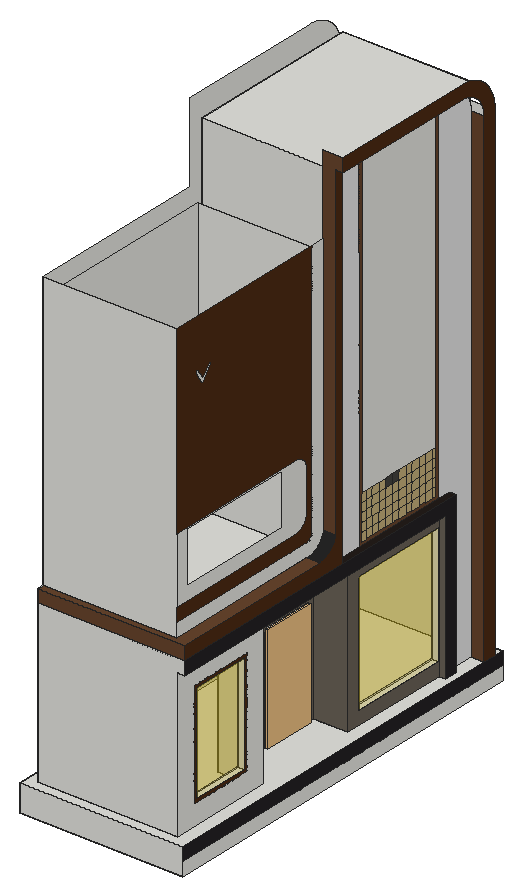
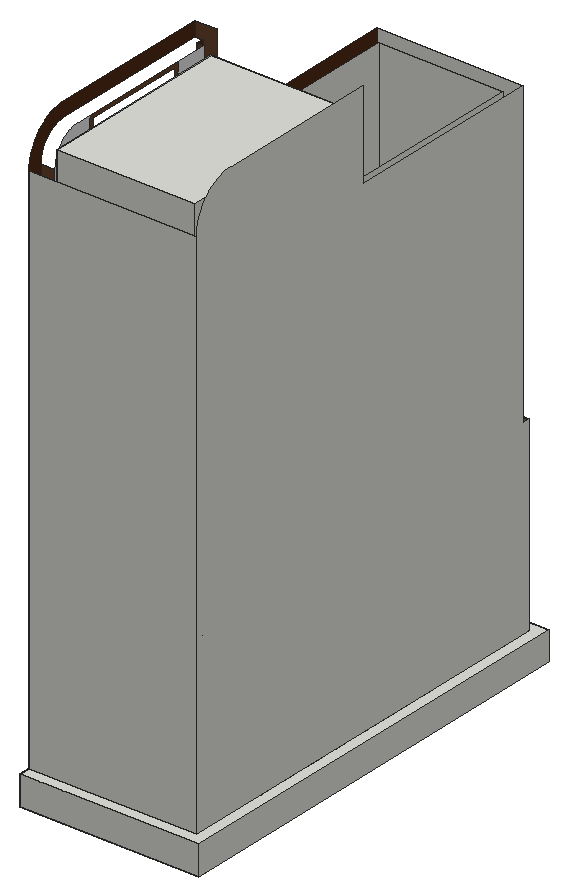
# SketchUp Ruby script. Lengths in inches.
U = 1.inch
M = Sketchup.active_model
def pt(a) = Geom::Point3d.new(a.map { |v| v * U })
def face(e, loops, mat)
  f = e.add_face(loops[0].map { |a| pt(a) })
  loops[1..].each { |l| e.add_face(l.map { |a| pt(a) }).erase! }
  f.material = f.back_material = mat if mat
  f
end
# faces: each face lists its corners as indices into pts; further lists are holes
def faces(e, pts, list, mat = nil) = list.each { |f| face(e, (f[0].is_a?(Array) ? f : [f]).map { |l| l.map { |i| pts[i] } }, mat) }
# xy, xz, yz: faces in a plane at the given z, y or x. An outline is a flat list of corners, or four numbers for a rectangle; further outlines are holes
def ring(l) = l.size == 4 ? [[l[0], l[1]], [l[2], l[1]], [l[2], l[3]], [l[0], l[3]]] : l.each_slice(2).to_a
def flat(e, list, mat, &to3) = list.each { |f| face(e, (f[0].is_a?(Array) ? f : [f]).map { |l| ring(l).map { |u, v| to3.(u, v) } }, mat) }
def xy(e, z, list, mat = nil) = flat(e, list, mat) { |x, y| [x, y, z] }
def xz(e, y, list, mat = nil) = flat(e, list, mat) { |x, z| [x, y, z] }
def yz(e, x, list, mat = nil) = flat(e, list, mat) { |y, z| [x, y, z] }
def lines(e, pts, list) = list.each { |a, b| e.add_line(pt(pts[a]), pt(pts[b])) }
# prism: a flat outline (further loops are holes) pulled along v
def prism(e, loops, v, mat = nil)
  f = face(e, loops, mat); d = Geom::Vector3d.new(v.map { |x| x * U })
  f.pushpull(f.normal.samedirection?(d) ? d.length : -d.length)
end
def box(e, o, s, mat = nil) = prism(e, [[o, [o[0] + s[0], o[1], o[2]], [o[0] + s[0], o[1] + s[1], o[2]], [o[0], o[1] + s[1], o[2]]]], [0, 0, s[2]], mat)
def at(x, y, z, deg = 0) = Geom::Transformation.translation(pt([x, y, z])) * Geom::Transformation.rotation(ORIGIN, Z_AXIS, deg.degrees)
def axes(o, x, y, z) = Geom::Transformation.new([*x, 0, *y, 0, *z, 0, *pt(o).to_a, 1])
def part(name) = M.definitions.add(name)
# library, detail: a bought-in or finely detailed component or shape, given as its bounding box
def library(name, o, s) = part(name).tap { |d| box(d.entities, o, s) }
def detail(e, o, s) = box(e.add_group.entities, o, s)
def put(e, d, t, mat = nil) = e.add_instance(d, t).tap { |i| i.material = mat if mat }
def group(e, t, mat = nil) = e.add_group.tap { |g| g.transformation = t; g.material = mat if mat }.entities
root = M.entities
M.materials.add("Glass_Basic_01").color = [255, 223, 26]
M.materials["Glass_Basic_01"].alpha = 0.25
M.materials.add("Marble_07_1K").color = [36, 34, 36]
M.materials.add("Metal_10_1K").color = [196, 175, 123]
M.materials.add("Plaster_04_1K").color = [106, 98, 87]
M.materials.add("Wood_Floor_12_1K").color = [35, 29, 25]
M.materials.add("Wood_Planks_01_1K").color = [69, 67, 63]
M.materials.add("Wood_Veneer_15_1K").color = [103, 69, 45]
M.materials.add("[Color_001]").color = [226, 226, 226]
M.materials.add("[Wood_Cherry_Original]1").color = [76, 43, 21]
c1 = library("porta+4",[0.2,-5.42,1.33],[46.55,4.72,83.21])
box(root,[15,186,177],[114,159,307.29])
xy(root,0,[[0,0,147,360]])
xy(root,24,[[0,0,147,0,147,339,135,339,135,315,141,315,141,303,135,303,135,201,103.5,201,103.5,105,135,105,135,9,9,9,9,351,147,351,147,360,0,360],[9,9,135,9,135,105,129,105,129,15,15,15,15,291,9,291],[15,15,129,15,129,99,99,99,99,207,129,207,129,345,15,345],[99,99,129,99,129,105,103.5,105,103.5,201,135,201,135,291,129,291,129,207,99,207],[9,291,15,291,15,345,129,345,129,291,135,291,135,339,147,339,147,351,9,351]])
xy(root,27,[[99,150,103.5,192]])
xy(root,36,[[129,213,135,303]])
xy(root,45,[[129,30,135,84]])
xy(root,117,[[99,150,103.5,192]])
xy(root,135,[[129,30,135,84]])
xy(root,144,[[129,213,135,303]])
xy(root,156,[[135,9,135,105,103.5,105,103.5,201,135,201,135,303,141,303,141,9]],"Plaster_04_1K")
xy(root,168,[[9,9,129,15],[15,15,15,345,129,345,129,207,99,207,99,99,129,99,129,15]])
xy(root,168,[[135,186,141,315]],"Wood_Floor_12_1K")
xy(root,177,[[21,21,123,174]])
xy(root,180,[[9,9,141,9,141,162,129,162,129,15,9,15],[129,162,141,162.25]],"Wood_Veneer_15_1K")
xz(root,0,[[0,0,147,24]])
xz(root,9,[[9,24,135,24,135,156,141,156,141,168,9,168]])
xz(root,9,[[9,168,141,180]],"Wood_Veneer_15_1K")
xz(root,15,[[15,24,129,168],[9,180,129,429]])
xz(root,21,[[21,177,123,423]])
xz(root,30,[[129,45,135,135]])
xz(root,84,[[129,45,135,135]])
xz(root,99,[[99,24,129,168]])
xz(root,105,[[103.5,24,135,156]])
xz(root,150,[[99,27,103.5,117]])
xz(root,174,[[21,177,123,423]])
xz(root,180,[[129,194.38,141,194.38,141,489,147,489,147,501,129,501]],"Wood_Veneer_15_1K")
xz(root,186,[[135,168,141,170],[135,170,141,170.38],[135,170.38,141,489]],"Wood_Veneer_15_1K")
xz(root,192,[[99,27,103.5,117]])
xz(root,201,[[103.5,24,135,156]],"Plaster_04_1K")
xz(root,207,[[99,24,129,168]])
xz(root,213,[[129,36,135,144]])
xz(root,303,[[129,36,135,144]])
xz(root,303,[[135,24,141,156]],"Plaster_04_1K")
xz(root,315,[[135,24,141,168]],"Wood_Floor_12_1K")
xz(root,339,[[135,24,147,465]],"Wood_Veneer_15_1K")
xz(root,345,[[15,24,129,168]])
xz(root,351,[[9,24,147,465]])
xz(root,360,[[0,0,147,24]])
yz(root,0,[[0,0,360,24]])
yz(root,9,[[9,24,9,180,15,180,15,429,180,429,180,501,315,501,316.13,500.98,317.26,500.93,318.39,500.84,319.51,500.72,320.63,500.56,321.75,500.36,322.85,500.13,323.95,499.87,325.04,499.57,326.125,499.24,327.19,498.87,328.25,498.47,329.3,498.04,330.33,497.57,331.34,497.08,332.34,496.55,333.33,495.99,334.29,495.4,335.24,494.77,336.16,494.125,337.06,493.45,337.95,492.74,338.81,492,339.64,491.24,340.46,490.46,341.24,489.64,342,488.81,342.74,487.95,343.45,487.06,344.125,486.16,344.77,485.24,345.4,484.29,345.99,483.33,346.55,482.34,347.08,481.34,347.57,480.33,348.04,479.3,348.47,478.25,348.87,477.19,349.24,476.125,349.57,475.04,349.87,473.95,350.13,472.85,350.36,471.75,350.56,470.63,350.72,469.51,350.84,468.39,350.93,467.26,350.98,466.13,351,465,351,24]])
yz(root,15,[[15,24,345,168]])
yz(root,21,[[21,177,174,423]])
yz(root,99,[[[99,24,207,168],[150,27,192,117]]])
yz(root,103.5,[[[147,24,195,120],[150,27,192,117]]])
yz(root,103.5,[[105,24,147,24,147,120,195,120,195,24,201,24,201,156,105,156]],"Plaster_04_1K")
yz(root,123,[[[21,177,174,423],[34,211,140.71,257]]])
yz(root,129,[[[15,24,99,168],[30,45,84,135]],[[207,24,345,168],[213,36,303,144]],[15,180,162.25,180,162.75,180.02,162.99,180.03,163.24,180.04,163.74,180.08,163.99,180.11,164.23,180.14,164.73,180.2,164.97,180.24,165.22,180.28,165.46,180.33,165.71,180.375,165.95,180.43,166.19,180.48,166.43,180.54,166.68,180.6,166.92,180.67,167.16,180.73,167.39,180.81,167.63,180.88,167.87,180.96,168.1,181.04,168.34,181.12,169.03,181.39,169.72,181.69,169.94,181.8,170.17,181.9,170.39,182.02,170.61,182.13,171.05,182.37,171.26,182.49,171.48,182.62,171.6875,182.75,171.9,182.88,172.11,183.01,172.32,183.15,172.52,183.29,172.73,183.4375,172.93,183.58,173.32,183.88,173.52,184.04,173.71,184.19,174.09,184.51,174.28,184.68,174.46,184.84,174.65,185.01,174.83,185.1875,175,185.36,175.35,185.71,175.52,185.9,175.69,186.08,175.86,186.27,176.02,186.45,176.18,186.64,176.34,186.84,176.49,187.03,176.65,187.23,176.8,187.42,176.94,187.625,177.09,187.83,177.23,188.03,177.51,188.45,177.9,189.08,178.02,189.3,178.14,189.51,178.38,189.95,178.49,190.17,178.6,190.4,178.71,190.62,178.8125,190.85,178.92,191.07,179.01,191.3,179.11,191.53,179.2,191.76,179.29,192,179.375,192.23,179.46,192.47,179.54,192.7,179.61,192.9375,179.68,193.18,179.75,193.41,179.82,193.65,179.88,193.9,180,194.38,180,429,168,429,168,196.07,167.98,196.03,167.95,195.95,167.92,195.875,167.88,195.79,167.85,195.72,167.73,195.48,167.6875,195.4,167.65,195.33,167.6,195.25,167.5625,195.18,167.52,195.1,167.47,195.03,167.42,194.95,167.33,194.81,167.18,194.6,167.07,194.46,167.02,194.39,166.96,194.32,166.9,194.26,166.85,194.19,166.79,194.125,166.49,193.8125,166.42,193.75,166.36,193.69,166.3,193.64,166.16,193.52,166.1,193.47,166.03,193.41,165.89,193.31,165.82,193.25,165.54,193.05,165.46,193.01,165.39,192.96,165.31,192.92,165.24,192.87,165.16,192.83,165.09,192.79,164.93,192.71,164.86,192.67,164.7,192.59,164.62,192.56,164.54,192.52,164.46,192.49,164.38,192.45,164.22,192.39,164.13,192.36,164.05,192.34,163.89,192.28,163.8,192.26,163.72,192.23,163.55,192.1875,163.47,192.17,163.38,192.15,163.3,192.13,163.21,192.11,163.125,192.1,163.04,192.08,162.95,192.07,162.87,192.06,162.69,192.04,162.61,192.03,162.43,192.01,162.26,192.01,162.17,192,15,192]])
yz(root,129,[[213,36,303,144],[30,45,84,135]],"Glass_Basic_01")
yz(root,129,[[[15,192,162.17,192,162.26,192.01,162.43,192.01,162.61,192.03,162.69,192.04,162.87,192.06,162.95,192.07,163.04,192.08,163.125,192.1,163.21,192.11,163.3,192.13,163.38,192.15,163.47,192.17,163.55,192.1875,163.72,192.23,163.8,192.26,163.89,192.28,164.05,192.34,164.13,192.36,164.22,192.39,164.38,192.45,164.46,192.49,164.54,192.52,164.62,192.56,164.7,192.59,164.86,192.67,164.93,192.71,165.09,192.79,165.16,192.83,165.24,192.87,165.31,192.92,165.39,192.96,165.46,193.01,165.54,193.05,165.82,193.25,165.89,193.31,166.03,193.41,166.1,193.47,166.16,193.52,166.3,193.64,166.36,193.69,166.42,193.75,166.49,193.8125,166.79,194.125,166.85,194.19,166.9,194.26,166.96,194.32,167.02,194.39,167.07,194.46,167.18,194.6,167.33,194.81,167.42,194.95,167.47,195.03,167.52,195.1,167.5625,195.18,167.6,195.25,167.65,195.33,167.6875,195.4,167.73,195.48,167.85,195.72,167.88,195.79,167.92,195.875,167.95,195.95,167.98,196.03,168,196.07,168,429,15,429,15,264,150.15,264,150.34,263.99,150.52,263.99,150.71,263.98,150.9,263.96,151.09,263.95,151.28,263.93,151.46,263.91,151.84,263.85,152.02,263.82,152.21,263.79,152.39,263.75,152.58,263.71,152.76,263.67,152.94,263.62,153.31,263.52,153.49,263.47,153.85,263.35,154.02,263.29,154.2,263.23,154.38,263.16,154.55,263.09,154.73,263.01,154.9,262.9375,155.07,262.86,155.24,262.78,155.41,262.69,155.57,262.61,155.74,262.52,155.91,262.42,156.07,262.33,156.55,262.03,156.7,261.92,156.86,261.82,157.16,261.6,157.3125,261.48,157.46,261.37,157.61,261.25,157.75,261.125,157.9,261,158.04,260.875,158.17,260.75,158.3125,260.62,158.44,260.49,158.58,260.35,158.71,260.21,158.84,260.08,158.96,259.9375,159.08,259.79,159.21,259.65,159.32,259.5,159.44,259.35,159.56,259.21,159.67,259.05,159.78,258.9,159.88,258.75,159.99,258.59,160.29,258.11,160.38,257.95,160.48,257.78,160.56,257.62,160.74,257.28,160.82,257.11,160.9,256.9375,160.97,256.77,161.05,256.59,161.12,256.42,161.18,256.24,161.25,256.06,161.3125,255.89,161.37,255.71,161.43,255.53,161.53,255.17,161.58,254.98,161.63,254.8,161.67,254.62,161.71,254.43,161.75,254.25,161.78,254.0625,161.8125,253.88,161.84,253.69,161.86,253.5,161.89,253.32,161.91,253.13,161.92,252.94,161.9375,252.75,161.95,252.57,161.95,252.375,161.96,252.1875,161.96,215.8125,161.95,215.625,161.95,215.43,161.9375,215.25,161.92,215.06,161.91,214.87,161.89,214.68,161.86,214.5,161.84,214.31,161.8125,214.12,161.78,213.9375,161.75,213.75,161.71,213.57,161.67,213.38,161.63,213.2,161.58,213.02,161.53,212.83,161.43,212.47,161.37,212.29,161.3125,212.11,161.25,211.94,161.18,211.76,161.12,211.58,161.05,211.41,160.97,211.23,160.9,211.0625,160.82,210.89,160.74,210.72,160.56,210.38,160.48,210.22,160.38,210.05,160.29,209.89,159.99,209.41,159.88,209.25,159.78,209.1,159.67,208.95,159.56,208.79,159.44,208.65,159.32,208.5,159.21,208.35,159.08,208.21,158.96,208.0625,158.84,207.92,158.71,207.79,158.58,207.65,158.44,207.51,158.3125,207.38,158.17,207.25,158.04,207.125,157.9,207,157.75,206.875,157.61,206.75,157.46,206.63,157.3125,206.52,157.16,206.4,156.86,206.18,156.7,206.08,156.55,205.97,156.07,205.67,155.91,205.58,155.74,205.48,155.57,205.39,155.41,205.31,155.24,205.22,155.07,205.14,154.9,205.0625,154.73,204.99,154.55,204.91,154.38,204.84,154.2,204.77,154.02,204.71,153.85,204.65,153.49,204.53,153.31,204.48,152.94,204.38,152.76,204.33,152.58,204.29,152.39,204.25,152.21,204.21,152.02,204.18,151.84,204.15,151.46,204.09,151.28,204.07,151.09,204.05,150.9,204.04,150.71,204.02,150.52,204.01,150.34,204.01,150.15,204,15,204],[45.07,371.33,42.96,374.22,43.02,374.3,36.28,383.51,36.24,383.87,36.27,384.22,36.36,384.57,36.52,384.89,36.74,385.17,37,385.41,37.3125,385.59,37.65,385.72,38,385.77,38.36,385.75,38.71,385.67,39.03,385.52,45.13,377.19,51.23,385.52,51.56,385.67,51.9,385.75,52.26,385.77,52.62,385.72,52.95,385.59,53.26,385.41,53.53,385.17,53.74,384.89,53.9,384.57,54,384.22,54.02,383.87,53.98,383.51,47.18,374.22,45.26,371.58]]],"[Wood_Cherry_Original]1")
yz(root,135,[[[9,24,105,156],[27,42,87,138]]])
yz(root,135,[[213,36,303,144],[30,45,84,135]],"Glass_Basic_01")
yz(root,135,[[216,171,220.5,178.875],[220.5,171,228,178.875],[228,171,235.5,178.875],[235.5,171,243,178.875],[243,171,250.5,178.875],
  [250.5,171,258,178.875],[258,171,265.5,178.875],[265.5,171,273,178.875],[273,171,280.5,178.875],[280.5,171,288,178.875],
  [288,171,295.5,178.875],[295.5,171,300,178.875],[216,178.875,220.5,186.75],[220.5,178.875,228,186.75],[228,178.875,235.5,186.75],
  [235.5,178.875,243,186.75],[243,178.875,250.5,186.75],[250.5,178.875,258,186.75],[258,178.875,265.5,186.75],[265.5,178.875,273,186.75],
  [273,178.875,280.5,186.75],[280.5,178.875,288,186.75],[288,178.875,295.5,186.75],[295.5,178.875,300,186.75],[216,186.75,220.5,194.625],
  [220.5,186.75,228,194.625],[228,186.75,235.5,194.625],[235.5,186.75,243,194.625],[243,186.75,250.5,194.625],[250.5,186.75,258,194.625],
  [258,186.75,265.5,194.625],[265.5,186.75,273,194.625],[273,186.75,280.5,194.625],[280.5,186.75,288,194.625],[288,186.75,295.5,194.625],
  [295.5,186.75,300,194.625],[216,194.625,220.5,202.5],[220.5,194.625,228,202.5],[228,194.625,235.5,202.5],[235.5,194.625,243,202.5],
  [243,194.625,250.5,202.5],[250.5,194.625,258,202.5],[258,194.625,265.5,202.5],[265.5,194.625,273,202.5],[273,194.625,280.5,202.5],
  [280.5,194.625,288,202.5],[288,194.625,295.5,202.5],[295.5,194.625,300,202.5],[216,202.5,220.5,210.375],[220.5,202.5,228,210.375],
  [228,202.5,235.5,210.375],[235.5,202.5,243,210.375],[258,202.5,265.5,210.375],[265.5,202.5,273,210.375],[273,202.5,280.5,210.375],
  [280.5,202.5,288,210.375],[288,202.5,295.5,210.375],[295.5,202.5,300,210.375]],"Metal_10_1K")
yz(root,135,[[201,24,303,24,303,36,213,36,213,144,303,144,303,156,201,156]],"Plaster_04_1K")
yz(root,135,[[243,202.5,250.5,210.375],[250.5,202.5,258,210.375]],"Wood_Planks_01_1K")
yz(root,135,[[[213,168,303,489],[216,171,300,486]]],"Wood_Veneer_15_1K")
yz(root,135,[[315,24,339,24,339,465,338.99,465.75,338.95,466.51,338.89,467.26,338.8125,468.01,338.7,468.75,338.57,469.5,338.42,470.24,338.25,470.97,338.05,471.7,337.83,472.42,337.58,473.13,337.31,473.83,337.03,474.53,336.72,475.22,336.38,475.9,336.03,476.5625,335.66,477.22,335.26,477.86,334.85,478.49,334.42,479.11,333.96,479.71,333.49,480.3,333,480.87,332.5,481.43,331.97,481.97,331.43,482.5,330.87,483,330.3,483.49,329.71,483.96,329.11,484.42,328.49,484.85,327.86,485.26,327.22,485.66,326.5625,486.03,325.9,486.38,325.22,486.72,324.53,487.03,323.83,487.31,323.13,487.58,322.42,487.83,321.7,488.05,320.97,488.25,320.24,488.42,319.5,488.57,318.75,488.7,318.01,488.8125,317.26,488.89,316.51,488.95,315.75,488.99,315,489,303,489,303,168,315,168],[186,168,213,489]],"[Color_001]")
yz(root,135,[[[27,42,87,138],[30,45,84,135]]],"[Wood_Cherry_Original]1")
yz(root,141,[[303,24,315,24,315,168,9,168,9,156,303,156]],"Marble_07_1K")
yz(root,141,[[9,168,186,168,186,489,180,489,180,194.38,179.88,193.9,179.82,193.65,179.75,193.41,179.68,193.18,179.61,192.9375,179.54,192.7,179.46,192.47,179.375,192.23,179.29,192,179.2,191.76,179.11,191.53,179.01,191.3,178.92,191.07,178.8125,190.85,178.71,190.62,178.6,190.4,178.49,190.17,178.38,189.95,178.14,189.51,178.02,189.3,177.9,189.08,177.51,188.45,177.23,188.03,177.09,187.83,176.94,187.625,176.8,187.42,176.65,187.23,176.49,187.03,176.34,186.84,176.18,186.64,176.02,186.45,175.86,186.27,175.69,186.08,175.52,185.9,175.35,185.71,175,185.36,174.83,185.1875,174.65,185.01,174.46,184.84,174.28,184.68,174.09,184.51,173.71,184.19,173.52,184.04,173.32,183.88,172.93,183.58,172.73,183.4375,172.52,183.29,172.32,183.15,172.11,183.01,171.9,182.88,171.6875,182.75,171.48,182.62,171.26,182.49,171.05,182.37,170.61,182.13,170.39,182.02,170.17,181.9,169.94,181.8,169.72,181.69,169.03,181.39,168.34,181.12,168.1,181.04,167.87,180.96,167.63,180.88,167.39,180.81,167.16,180.73,166.92,180.67,166.68,180.6,166.43,180.54,166.19,180.48,165.95,180.43,165.71,180.375,165.46,180.33,165.22,180.28,164.97,180.24,164.73,180.2,164.23,180.14,163.99,180.11,163.74,180.08,163.24,180.04,162.99,180.03,162.75,180.02,162.25,180,9,180]],"[Wood_Cherry_Original]1")
yz(root,147,[[0,0,360,12]])
yz(root,147,[[0,12,360,24]],"Marble_07_1K")
yz(root,147,[[339,24,351,24,351,465,350.98,466.13,350.93,467.26,350.84,468.39,350.72,469.51,350.56,470.63,350.36,471.75,350.13,472.85,349.87,473.95,349.57,475.04,349.24,476.125,348.87,477.19,348.47,478.25,348.04,479.3,347.57,480.33,347.08,481.34,346.55,482.34,345.99,483.33,345.4,484.29,344.77,485.24,344.125,486.16,343.45,487.06,342.74,487.95,342,488.81,341.24,489.64,340.46,490.46,339.64,491.24,338.81,492,337.95,492.74,337.06,493.45,336.16,494.125,335.24,494.77,334.29,495.4,333.33,495.99,332.34,496.55,331.34,497.08,330.33,497.57,329.3,498.04,328.25,498.47,327.19,498.87,326.125,499.24,325.04,499.57,323.95,499.87,322.85,500.13,321.75,500.36,320.63,500.56,319.51,500.72,318.39,500.84,317.26,500.93,316.13,500.98,315,501,180,501,180,489,315,489,315.75,488.99,316.51,488.95,317.26,488.89,318.01,488.8125,318.75,488.7,319.5,488.57,320.24,488.42,320.97,488.25,321.7,488.05,322.42,487.83,323.13,487.58,323.83,487.31,324.53,487.03,325.22,486.72,325.9,486.38,326.5625,486.03,327.22,485.66,327.86,485.26,328.49,484.85,329.11,484.42,329.71,483.96,330.3,483.49,330.87,483,331.43,482.5,331.97,481.97,332.5,481.43,333,480.87,333.49,480.3,333.96,479.71,334.42,479.11,334.85,478.49,335.26,477.86,335.66,477.22,336.03,476.5625,336.38,475.9,336.72,475.22,337.03,474.53,337.31,473.83,337.58,473.13,337.83,472.42,338.05,471.7,338.25,470.97,338.42,470.24,338.57,469.5,338.7,468.75,338.8125,468.01,338.89,467.26,338.95,466.51,338.99,465.75,339,465]],"[Wood_Cherry_Original]1")
p = [[129,162.25,180],[141,162.25,180],[141,162.5,180.01],[129,162.5,180.01],[141,162.75,180.02],[129,162.75,180.02],
  [141,162.99,180.03],[129,162.99,180.03],[141,163.24,180.04],[129,163.24,180.04],[141,163.49,180.06],[129,163.49,180.06],
  [141,163.74,180.08],[129,163.74,180.08],[141,163.99,180.11],[129,163.99,180.11],[141,164.23,180.14],[129,164.23,180.14],
  [141,164.48,180.17],[129,164.48,180.17],[141,164.73,180.2],[129,164.73,180.2],[141,164.97,180.24],[129,164.97,180.24],
  [141,165.22,180.28],[129,165.22,180.28],[141,165.46,180.33],[129,165.46,180.33],[141,165.71,180.375],[129,165.71,180.375],
  [141,165.95,180.43],[129,165.95,180.43],[141,166.19,180.48],[129,166.19,180.48],[141,166.43,180.54],[129,166.43,180.54],
  [141,166.68,180.6],[129,166.68,180.6],[141,166.92,180.67],[129,166.92,180.67],[141,167.16,180.73],[129,167.16,180.73],
  [141,167.39,180.81],[129,167.39,180.81],[141,167.63,180.88],[129,167.63,180.88],[141,167.87,180.96],[129,167.87,180.96],
  [141,168.1,181.04],[129,168.1,181.04],[141,168.34,181.12],[129,168.34,181.12],[141,168.57,181.21],[129,168.57,181.21],
  [141,168.8,181.3],[129,168.8,181.3],[141,169.03,181.39],[129,169.03,181.39],[141,169.26,181.49],[129,169.26,181.49],
  [141,169.49,181.59],[129,169.49,181.59],[141,169.72,181.69],[129,169.72,181.69],[141,169.94,181.8],[129,169.94,181.8],
  [141,170.17,181.9],[129,170.17,181.9],[141,170.39,182.02],[129,170.39,182.02],[141,170.61,182.13],[129,170.61,182.13],
  [141,170.83,182.25],[129,170.83,182.25],[141,171.05,182.37],[129,171.05,182.37],[141,171.26,182.49],[129,171.26,182.49],
  [141,171.48,182.62],[129,171.48,182.62],[141,171.6875,182.75],[129,171.6875,182.75],[141,171.9,182.88],[129,171.9,182.88],
  [141,172.11,183.01],[129,172.11,183.01],[141,172.32,183.15],[129,172.32,183.15],[141,172.52,183.29],[129,172.52,183.29],
  [141,172.73,183.4375],[129,172.73,183.4375],[141,172.93,183.58],[129,172.93,183.58],[141,173.125,183.73],[129,173.125,183.73],
  [141,173.32,183.88],[129,173.32,183.88],[141,173.52,184.04],[129,173.52,184.04],[141,173.71,184.19],[129,173.71,184.19],
  [141,173.9,184.35],[129,173.9,184.35],[141,174.09,184.51],[129,174.09,184.51],[141,174.28,184.68],[129,174.28,184.68],
  [141,174.46,184.84],[129,174.46,184.84],[141,174.65,185.01],[129,174.65,185.01],[141,174.83,185.1875],[129,174.83,185.1875],
  [141,175,185.36],[129,175,185.36],[141,175.18,185.54],[129,175.18,185.54],[141,175.35,185.71],[129,175.35,185.71],
  [141,175.52,185.9],[129,175.52,185.9],[141,175.69,186.08],[129,175.69,186.08],[141,175.86,186.27],[129,175.86,186.27],
  [141,176.02,186.45],[129,176.02,186.45],[141,176.18,186.64],[129,176.18,186.64],[141,176.34,186.84],[129,176.34,186.84],
  [141,176.49,187.03],[129,176.49,187.03],[141,176.65,187.23],[129,176.65,187.23],[141,176.8,187.42],[129,176.8,187.42],
  [141,176.94,187.625],[129,176.94,187.625],[141,177.09,187.83],[129,177.09,187.83],[141,177.23,188.03],[129,177.23,188.03],
  [141,177.37,188.24],[129,177.37,188.24],[141,177.51,188.45],[129,177.51,188.45],[141,177.64,188.66],[129,177.64,188.66],
  [141,177.77,188.87],[129,177.77,188.87],[141,177.9,189.08],[129,177.9,189.08],[141,178.02,189.3],[129,178.02,189.3],
  [141,178.14,189.51],[129,178.14,189.51],[141,178.26,189.73],[129,178.26,189.73],[141,178.38,189.95],[129,178.38,189.95],
  [141,178.49,190.17],[129,178.49,190.17],[141,178.6,190.4],[129,178.6,190.4],[141,178.71,190.62],[129,178.71,190.62],
  [141,178.8125,190.85],[129,178.8125,190.85],[141,178.92,191.07],[129,178.92,191.07],[141,179.01,191.3],[129,179.01,191.3],
  [141,179.11,191.53],[129,179.11,191.53],[141,179.2,191.76],[129,179.2,191.76],[141,179.29,192],[129,179.29,192],
  [141,179.375,192.23],[129,179.375,192.23],[141,179.46,192.47],[129,179.46,192.47],[141,179.54,192.7],[129,179.54,192.7],
  [141,179.61,192.9375],[129,179.61,192.9375],[141,179.68,193.18],[129,179.68,193.18],[141,179.75,193.41],[129,179.75,193.41],
  [141,179.82,193.65],[129,179.82,193.65],[141,179.88,193.9],[129,179.88,193.9],[141,179.94,194.14],[129,179.94,194.14],
  [141,180,194.38],[129,180,194.38],[9,291,0],[9,291,24],[9,9,0],[9,9,24],
  [15,345,168],[9,345,168],[129,99,168],[129,105,168],[129,180,180],[135,180,180],
  [129,162,180]]
faces(root,p,[[0,1,2,3],[3,2,4,5],[5,4,6,7],[7,6,8,9],[9,8,10,11],[11,10,12,13],[13,12,14,15],[15,14,16,17],
  [17,16,18,19],[19,18,20,21],[21,20,22,23],[23,22,24,25],[25,24,26,27],[27,26,28,29],[29,28,30,31],[31,30,32,33],
  [33,32,34,35],[35,34,36,37],[37,36,38,39],[39,38,40,41],[41,40,42,43],[43,42,44,45],[45,44,46,47],[47,46,48,49],
  [49,48,50,51],[51,50,52,53],[53,52,54,55],[55,54,56,57],[57,56,58,59],[59,58,60,61],[61,60,62,63],[63,62,64,65],
  [65,64,66,67],[67,66,68,69],[69,68,70,71],[71,70,72,73],[73,72,74,75],[75,74,76,77],[77,76,78,79],[79,78,80,81],
  [81,80,82,83],[83,82,84,85],[85,84,86,87],[87,86,88,89],[89,88,90,91],[91,90,92,93],[93,92,94,95],[95,94,96,97],
  [97,96,98,99],[99,98,100,101],[101,100,102,103],[103,102,104,105],[105,104,106,107],[107,106,108,109],[109,108,110,111],[111,110,112,113],
  [113,112,114,115],[115,114,116,117],[117,116,118,119],[119,118,120,121],[121,120,122,123],[123,122,124,125],[125,124,126,127],[127,126,128,129],
  [129,128,130,131],[131,130,132,133],[133,132,134,135],[135,134,136,137],[137,136,138,139],[139,138,140,141],[141,140,142,143],[143,142,144,145],
  [145,144,146,147],[147,146,148,149],[149,148,150,151],[151,150,152,153],[153,152,154,155],[155,154,156,157],[157,156,158,159],[159,158,160,161],
  [161,160,162,163],[163,162,164,165],[165,164,166,167],[167,166,168,169],[169,168,170,171],[171,170,172,173],[173,172,174,175],[175,174,176,177],
  [177,176,178,179],[179,178,180,181],[181,180,182,183],[183,182,184,185],[185,184,186,187],[187,186,188,189],[189,188,190,191],[191,190,192,193],
  [193,192,194,195],[195,194,196,197],[197,196,198,199]],"Wood_Veneer_15_1K")
lines(root,p,[[200,201],[202,203],[204,205],[206,207],[208,199],[209,208],[210,208]])
put(root,c1,axes([100.74,146.79,22.46],[0,1.03118,0],[-1,0,0],[0,0,1.15408]))
